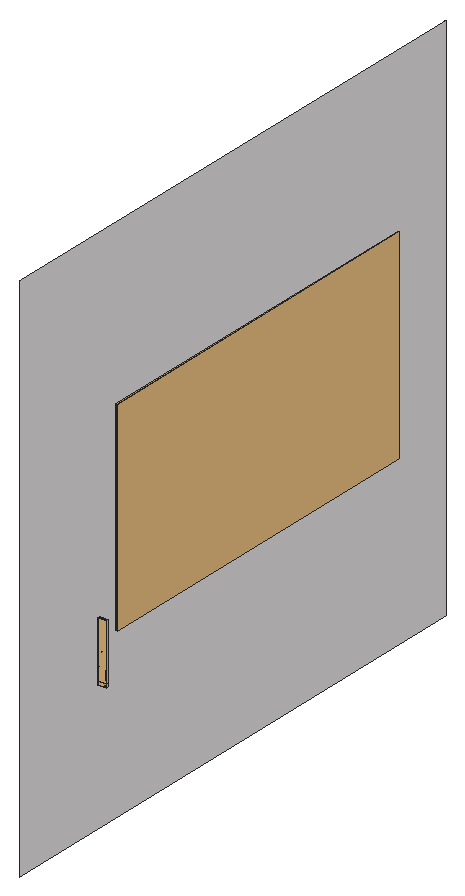
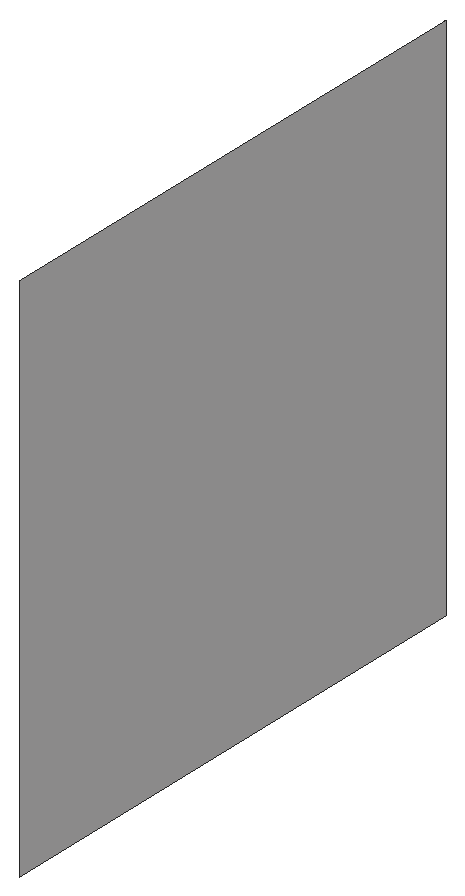
# SketchUp Ruby script. Lengths in inches.
U = 1.inch
M = Sketchup.active_model
def pt(a) = Geom::Point3d.new(a.map { |v| v * U })
def face(e, loops, mat)
  f = e.add_face(loops[0].map { |a| pt(a) })
  loops[1..].each { |l| e.add_face(l.map { |a| pt(a) }).erase! }
  f.material = f.back_material = mat if mat
  f
end
# faces: each face lists its corners as indices into pts; further lists are holes
def faces(e, pts, list, mat = nil) = list.each { |f| face(e, (f[0].is_a?(Array) ? f : [f]).map { |l| l.map { |i| pts[i] } }, mat) }
# xy, xz, yz: faces in a plane at the given z, y or x. An outline is a flat list of corners, or four numbers for a rectangle; further outlines are holes
def ring(l) = l.size == 4 ? [[l[0], l[1]], [l[2], l[1]], [l[2], l[3]], [l[0], l[3]]] : l.each_slice(2).to_a
def flat(e, list, mat, &to3) = list.each { |f| face(e, (f[0].is_a?(Array) ? f : [f]).map { |l| ring(l).map { |u, v| to3.(u, v) } }, mat) }
def xy(e, z, list, mat = nil) = flat(e, list, mat) { |x, y| [x, y, z] }
def xz(e, y, list, mat = nil) = flat(e, list, mat) { |x, z| [x, y, z] }
def yz(e, x, list, mat = nil) = flat(e, list, mat) { |y, z| [x, y, z] }
def lines(e, pts, list) = list.each { |a, b| e.add_line(pt(pts[a]), pt(pts[b])) }
# prism: a flat outline (further loops are holes) pulled along v
def prism(e, loops, v, mat = nil)
  f = face(e, loops, mat); d = Geom::Vector3d.new(v.map { |x| x * U })
  f.pushpull(f.normal.samedirection?(d) ? d.length : -d.length)
end
def box(e, o, s, mat = nil) = prism(e, [[o, [o[0] + s[0], o[1], o[2]], [o[0] + s[0], o[1] + s[1], o[2]], [o[0], o[1] + s[1], o[2]]]], [0, 0, s[2]], mat)
def at(x, y, z, deg = 0) = Geom::Transformation.translation(pt([x, y, z])) * Geom::Transformation.rotation(ORIGIN, Z_AXIS, deg.degrees)
def axes(o, x, y, z) = Geom::Transformation.new([*x, 0, *y, 0, *z, 0, *pt(o).to_a, 1])
def part(name) = M.definitions.add(name)
# library, detail: a bought-in or finely detailed component or shape, given as its bounding box
def library(name, o, s) = part(name).tap { |d| box(d.entities, o, s) }
def detail(e, o, s) = box(e.add_group.entities, o, s)
def put(e, d, t, mat = nil) = e.add_instance(d, t).tap { |i| i.material = mat if mat }
def group(e, t, mat = nil) = e.add_group.tap { |g| g.transformation = t; g.material = mat if mat }.entities
root = M.entities
M.materials.add("[Stone Vein Gray]").color = [225, 223, 223]
M.materials.add("green").color = [174, 139, 102]
M.materials.add("vio").color = [206, 114, 100]
c1 = library("3DGeom~133_Defintion",[-19.91,-529.75,-72.32],[39.82,1000,144.37])
c2 = library("3DGeom~131_Defintion",[-19.41,-483.5625,-70.5],[38.82,1000,140.74])
c3 = part("3DGeom~134_Defintion")
p = [[-9.17,365.0625,-60.44],[-10.66,319.24,-60.24],[-9.24,319.23,-61.125],[-10.63,365.04,-59.53],[-12.34,365.04,-59.02],[-14.12,365.04,-58.98],
  [-14.05,319.22,-59.71],[-12.32,319.23,-59.75],[-8.56,277.89,-58.6875],[-8.45,241.12,-52.31],[-7.11,241.05,-53.13],[-9.93,277.92,-57.83],
  [-11.54,277.92,-57.36],[-13.22,277.89,-57.32],[-11.63,241.07,-51.81],[-10.01,241.13,-51.85],[-6.75,470.15,-49.68],[-9.84,415.33,-55.7],
  [-8.34,415.37,-56.63],[-8.29,470.08,-48.72],[-10.1,470.07,-48.1875],[-13.43,415.34,-55.13],[-11.6,415.32,-55.17],[-11.98,470.11,-48.14],
  [-4.1,211.43,-41.85],[-0.64,188.37,-23.41],[0.67,188.13,-24.11],[-5.42,211.6,-41.08],[-6.95,211.62,-40.63],[-8.53,211.47,-40.56],
  [-3.6875,188.18,-22.85],[-2.14,188.39,-22.97],[6.29,168.75,-2.9375],[10.49,151.32,19.02],[11.76,151.06,18.38],[6.29,168.75,-2.9375],
  [4.99,169.02,-2.29],[10.49,151.32,19.02],[3.51,169.05,-1.87],[2,168.82,-1.72],[7.55,151.14,19.55],[9.03,151.35,19.42],
  [-2.58,-7.65,9.24],[-5.6,-27.13,7.79],[-4.52,-27.2,7.15],[-3.69,-7.65,9.88],[-4.97,-7.58,10.22],[-6.28,-7.43,10.23],
  [-8.15,-27.06,8.11],[-6.85,-27.08,8.125],[-3.875,-43.53,12.625],[-2.45,-57.47,24.41],[-1.39,-57.67,23.87],[-4.94,-43.36,13.22],
  [-6.17,-43.32,13.55],[-7.45,-43.42,13.58],[-4.9,-57.59,24.83],[-3.66,-57.4375,24.75],[7.01,37.63,28.93],[0.5,14.23,18.1875],
  [1.64,14.26,17.55],[5.85,37.59,29.58],[4.53,37.68,29.94],[-2.125,14.51,18.57],[-0.8,14.3125,18.55],[3.18,37.89,29.97],
  [5.56,-294.46,30.13],[4.07,-328.71,26.72],[4.85,-328.71,26.23],[4.75,-294.51,30.64],[4.86,-362.1,26.86],[4.11,-362.08,27.33],
  [4.47,-395.52,30.27],[5.1875,-395.55,29.82],[3.8,-294.53,30.93],[2.8125,-294.51,30.96],[2.21,-328.71,27.03],[3.16,-328.71,27],
  [3.23,-362.08,27.6],[2.32,-362.08,27.63],[2.75,-395.51,30.56],[3.63,-395.5,30.53],[5.84,-429.05,35.11],[6.16,-462.54,43.14],
  [6.82,-462.6,42.73],[5.15,-429,35.54],[4.35,-428.98,35.79],[3.51,-428.99,35.8125],[4.58,-462.53,43.4],[5.39,-462.51,43.375],
  [16.05,132.58,36.39],[16.75,110.79,47.79],[17.95,110.68,47.08],[14.8125,132.8,37.06],[13.38,132.84,37.45],[11.91,132.69,37.51],
  [13.89,110.82,48.16],[15.34,110.84,48.16],[2.27,-71.39,38.47],[5.25,-86.23,54.01],[6.27,-86.4,53.46],[1.23,-71.18,39],
  [8.9,-222.87,50.33],[6.22,-258.8,39.57],[7.0625,-258.72,39.05],[0.04,-71.16,39.34],[-1.17,-71.33,39.4375],[2.89,-86.37,54.44],
  [4.09,-86.22,54.36],[8.03,-222.96,50.86],[7.01,-223,51.17],[5.95,-222.97,51.21],[4.22,-258.8,39.9],[5.24,-258.83,39.86],
  [16.42,86.25,47.3],[11.16,61.76,40.67],[12.34,61.78,40],[15.23,86.27,48],[13.86,86.35,48.37],[8.43,62.04,41.06],
  [9.8125,61.85,41.04],[12.44,86.47,48.36],[8.12,-496.2,52.69],[9.15,-529.77,65.34],[9.75,-529.85,64.98],[7.49,-496.125,53.08],
  [6.76,-496.1,53.3],[5.99,-496.12,53.32],[7.72,-529.76,65.58],[8.45,-529.74,65.55],[11.66,-156.24,69.3],[9.6875,-188.37,61.86],
  [10.59,-188.28,61.31],[10.73,-156.3,69.88],[9.64,-156.33,70.21],[8.51,-156.32,70.24],[7.54,-188.38,62.22],[8.64,-188.4,62.18],
  [9.71,-104.66,65.64],[8.72,-104.5625,66.23],[10.65,-127.92,72.15],[11.61,-127.92,71.55],[7.58,-104.56,66.57],[6.4,-104.66,66.625],
  [8.36,-127.96,72.52],[9.53,-127.93,72.49]]
faces(c3.entities,p,[[0,1,2],[0,3,1],[4,5,6],[4,6,7],[8,9,10],[8,11,9],[12,13,14],[12,14,15],
  [16,17,18],[16,19,17],[20,21,22],[20,23,21],[24,25,26],[24,27,25],[28,29,30],[28,30,31],
  [32,33,34],[35,36,37],[38,39,40],[38,40,41],[42,43,44],[42,45,43],[46,47,48],[46,48,49],
  [50,51,52],[50,53,51],[54,55,56],[54,56,57],[58,59,60],[58,61,59],[62,63,64],[62,65,63],
  [66,67,68],[66,69,67],[70,71,72],[70,72,73],[74,75,76],[74,76,77],[78,79,80],[78,80,81],
  [82,83,84],[82,85,83],[86,87,88],[86,88,89],[90,91,92],[90,93,91],[94,95,96],[94,96,97],
  [98,99,100],[98,101,99],[102,103,104],[105,106,107],[105,107,108],[102,109,103],[110,111,112],[110,112,113],
  [114,115,116],[114,117,115],[118,119,120],[118,121,119],[122,123,124],[122,125,123],[126,127,128],[126,128,129],
  [130,131,132],[130,133,131],[134,135,136],[134,136,137],[138,139,140],[138,140,141],[142,143,144],[142,144,145]],"green")
c4 = part("3DGeom~132_Defintion")
p = [[-9.01,311.27,-59.6],[-10.4,311.27,-58.74],[-9.6875,270.99,-56.39],[-8.34,270.95,-57.22],[-8.13,405.01,-55.22],[-10.37,355.9375,-58.05],
  [-8.94,355.96,-58.93],[-12.01,311.27,-58.26],[-13.69,311.26,-58.22],[-12.89,270.96,-55.89],[-11.25,270.99,-55.92],[-9.6,404.97,-54.31],
  [-11.31,404.95,-53.8],[-13.77,355.9375,-57.51],[-12.03,355.93,-57.55],[-13.1,404.98,-53.75],[-6.9375,235.04,-51.81],[-5.28,206.32,-40.06],
  [-3.99,206.16,-40.81],[-8.24,235.11,-51],[-9.76,235.11,-50.55],[-11.34,235.05,-50.51],[-8.32,206.19,-39.54],[-6.77,206.34,-39.62],
  [-4.28,516.18,-38.61],[-8.09,458.36,-47.51],[-6.58,458.42,-48.44],[-5.83,516.1,-37.65],[-7.64,516.08,-37.11],[-11.68,458.38,-46.9375],
  [-9.85,458.34,-46.98],[-9.53,516.13,-37.0625],[0.66,183.44,-23.51],[4.86,164.8,-2.23],[6.13,164.54,-2.87],[-0.625,183.67,-22.83],
  [-2.09,183.69,-22.4],[-3.59,183.49,-22.28],[1.95,164.61,-1.68],[3.42,164.83,-1.82],[-4.41,-26.52,6.97],[-4.82,-42.28,12.89],
  [-3.78,-42.44,12.31],[-5.46,-26.45,7.59],[-6.68,-26.4,7.92],[-7.95,-26.38,7.91],[-7.26,-42.34,13.24],[-6.02,-42.24,13.21],
  [1.59,13.9,17.11],[-3.6,-7.46,9.63],[-2.52,-7.46,9.01],[0.49,13.87,17.73],[-0.78,13.96,18.08],[-6.12,-7.25,9.97],
  [-4.84,-7.39,9.97],[-2.07,14.15,18.11],[11.47,147.29,17.92],[14.44,129.49,36.13],[15.65,129.27,35.48],[11.47,147.29,17.92],
  [10.22,147.54,18.54],[8.81,147.58,18.9375],[7.36,147.375,19.06],[11.62,129.38,36.57],[13.05,129.53,36.51],[-1.35,-56.24,23.27],
  [1.2,-69.4,38.03],[2.21,-69.6,37.51],[-2.38,-56.03,23.8],[-3.5625,-56,24.13],[-4.77,-56.16,24.21],[-1.15,-69.55,38.45],
  [0.04,-69.38,38.36],[4.73,-320.51,25.58],[3.97,-320.51,26.06],[4.01,-353.05,26.65],[4.74,-353.07,26.19],[3.08,-320.51,26.33],
  [2.15,-320.51,26.36],[2.26,-353.05,26.94],[3.15,-353.05,26.91],[12.03,60.24,39],[5.7,36.65,28.84],[6.83,36.6875,28.21],
  [10.88,60.22,39.65],[5.06,-385.68,29.08],[4.36,-385.65,29.52],[5.02,-418.3,34.66],[5.7,-418.34,34.23],[9.57,60.3,40.01],
  [3.1,36.95,29.23],[4.41,36.74,29.2],[8.22,60.49,40.03],[6.89,-252.26,38.07],[4.63,-287.17,29.875],[5.42,-287.12,29.38],
  [3.54,-385.64,29.77],[2.68,-385.64,29.79],[3.42,-418.29,34.92],[4.24,-418.28,34.89],[6.07,-252.34,38.58],[5.11,-252.37,38.87],
  [4.11,-252.34,38.9],[2.74,-287.17,30.1875],[3.71,-287.19,30.16],[6.65,-451.06,41.67],[7.3,-483.75,51.75],[7.92,-483.82,51.375],
  [6.01,-451,42.07],[5.26,-450.97,42.29],[4.47,-450.99,42.32],[5.84,-483.74,51.99],[6.59,-483.72,51.97],[17.5,107.92,45.9],
  [16.33,108.02,46.59],[14.85,84.12,46.8],[16.01,84.1,46.12],[14.96,108.07,46.96],[12.125,84.32,47.16],[13.51,84.19,47.16],
  [13.54,108.06,46.96],[10.32,-183.58,59.78],[7.83,-217.4,49.6],[8.67,-217.31,49.07],[9.44,-183.67,60.32],[8.42,-183.7,60.63],
  [7.35,-183.68,60.66],[5.8,-217.4,49.93],[6.83,-217.43,49.89],[6.11,-84.25,52.125],[8.51,-101.95,64.58],[9.47,-102.05,64],
  [5.12,-84.08,52.67],[3.99,-84.07,53],[2.82,-84.22,53.08],[6.24,-102.05,64.96],[7.39,-101.95,64.91],[11.32,-124.73,69.76],
  [10.46,-152.4,68.13],[11.37,-152.34,67.57],[10.39,-124.73,70.35],[9.3,-124.74,70.69],[8.15,-124.76,70.71],[8.29,-152.42,68.49],
  [9.4,-152.43,68.46]]
faces(c4.entities,p,[[0,1,2],[0,2,3],[4,5,6],[7,8,9],[7,9,10],[4,11,5],[12,13,14],[12,15,13],
  [16,17,18],[16,19,17],[20,21,22],[20,22,23],[24,25,26],[24,27,25],[28,29,30],[28,31,29],
  [32,33,34],[32,35,33],[36,37,38],[36,38,39],[40,41,42],[40,43,41],[44,45,46],[44,46,47],
  [48,49,50],[48,51,49],[52,53,54],[52,55,53],[56,57,58],[59,60,57],[61,62,63],[61,63,64],
  [65,66,67],[65,68,66],[69,70,71],[69,71,72],[73,74,75],[73,75,76],[77,78,79],[77,79,80],
  [81,82,83],[81,84,82],[85,86,87],[85,87,88],[89,90,91],[89,92,90],[93,94,95],[96,97,98],
  [96,98,99],[93,100,94],[101,102,103],[101,103,104],[105,106,107],[105,108,106],[109,110,111],[109,111,112],
  [113,114,115],[113,115,116],[117,118,119],[117,120,118],[121,122,123],[121,124,122],[125,126,127],[125,127,128],
  [129,130,131],[129,132,130],[133,134,135],[133,135,136],[137,138,139],[137,140,138],[141,142,143],[141,143,144]],"green")
c5 = part("3DGeom~130_Defintion")
p = [[-10.63,365.1,-59.54],[-12.32,319.28,-59.76],[-10.66,319.28,-60.25],[-12.34,365.09,-59.03],[-9.9375,277.96,-57.84],[-11.54,277.96,-57.36],
  [-10.01,241.16,-51.85],[-8.45,241.16,-52.32],[-8.3,470.15,-48.73],[-11.6,415.375,-55.18],[-9.85,415.39,-55.7],[-10.1,470.14,-48.19],
  [-5.42,211.63,-41.09],[-6.95,211.65,-40.64],[-2.14,188.42,-22.97],[-0.64,188.4,-23.41],[4.99,169.04,-2.29],[9.03,151.375,19.43],
  [10.49,151.34,19.02],[3.51,169.07,-1.87],[-3.69,-7.65,9.88],[-6.85,-27.08,8.125],[-5.6,-27.13,7.79],[-4.97,-7.58,10.23],
  [-4.94,-43.37,13.22],[-3.66,-57.45,24.75],[-2.45,-57.48,24.42],[-6.18,-43.33,13.55],[5.85,37.6,29.58],[-0.8,14.32,18.55],
  [0.5,14.23,18.19],[4.53,37.6875,29.95],[4.75,-294.56,30.64],[3.16,-328.76,27.01],[4.07,-328.76,26.73],[3.8,-294.58,30.93],
  [4.11,-362.14,27.34],[3.23,-362.13,27.61],[3.63,-395.56,30.53],[4.47,-395.57,30.28],[5.15,-429.0625,35.55],[4.35,-429.04,35.79],
  [5.39,-462.58,43.38],[6.16,-462.6,43.15],[14.8125,132.82,37.06],[15.35,110.85,48.17],[16.75,110.8,47.79],[13.39,132.86,37.45],
  [1.23,-71.19,39],[0.04,-71.17,39.34],[4.09,-86.23,54.36],[5.25,-86.24,54.02],[8.03,-222.99,50.87],[5.24,-258.86,39.87],
  [6.22,-258.83,39.57],[7.01,-223.03,51.18],[15.23,86.29,48],[9.81,61.86,41.04],[11.16,61.77,40.67],[13.86,86.36,48.375],
  [7.49,-496.2,53.08],[6.76,-496.17,53.3],[8.45,-529.82,65.5625],[9.15,-529.85,65.35],[10.73,-156.33,69.89],[8.64,-188.43,62.1875],
  [9.6875,-188.39,61.87],[9.64,-156.35,70.22],[8.73,-104.58,66.24],[7.58,-104.57,66.58],[9.53,-127.95,72.5],[10.66,-127.9375,72.16]]
faces(c5.entities,p,[[0,1,2],[0,3,1],[4,5,6],[4,6,7],[8,9,10],[8,11,9],[12,13,14],[12,14,15],
  [16,17,18],[16,19,17],[20,21,22],[20,23,21],[24,25,26],[24,27,25],[28,29,30],[28,31,29],
  [32,33,34],[32,35,33],[36,37,38],[36,38,39],[40,41,42],[40,42,43],[44,45,46],[44,47,45],
  [48,49,50],[48,50,51],[52,53,54],[52,55,53],[56,57,58],[56,59,57],[60,61,62],[60,62,63],
  [64,65,66],[64,67,65],[68,69,70],[68,70,71]],"green")
c6 = part("3DGeom~129_Defintion")
p = [[-10.4,311.32,-58.75],[-12.01,311.32,-58.27],[-11.25,271.03,-55.93],[-9.6875,271.03,-56.4],[-9.6,405.03,-54.31],[-12.03,355.98,-57.5625],
  [-10.37,355.99,-58.06],[-11.3125,405.02,-53.8],[-8.24,235.14,-51.01],[-9.76,235.15,-50.5625],[-6.78,206.37,-39.62],[-5.28,206.35,-40.0625],
  [-5.83,516.18,-37.66],[-9.85,458.41,-46.99],[-8.09,458.42,-47.52],[-7.64,516.16,-37.12],[-0.625,183.7,-22.83],[3.42,164.86,-1.82],
  [4.87,164.83,-2.23],[-2.09,183.72,-22.4],[-5.46,-26.46,7.59],[-6.68,-26.41,7.92],[-6.02,-42.25,13.22],[-4.82,-42.29,12.89],
  [0.49,13.875,17.74],[-4.84,-7.39,9.97],[-3.6,-7.46,9.63],[-0.78,13.96,18.09],[10.23,147.57,18.54],[8.81,147.6,18.94],
  [13.05,129.54,36.52],[14.44,129.5,36.14],[-2.39,-56.04,23.81],[-3.56,-56.01,24.13],[0.04,-69.39,38.36],[1.2,-69.42,38.03],
  [3.97,-320.56,26.0625],[3.08,-320.5625,26.33],[3.15,-353.1,26.92],[4.01,-353.11,26.65],[10.88,60.23,39.66],[4.41,36.75,29.2],
  [5.7,36.66,28.85],[9.57,60.3125,40.02],[4.36,-385.71,29.52],[4.24,-418.34,34.9],[5.02,-418.36,34.66],[3.54,-385.69,29.77],
  [6.07,-252.38,38.58],[3.71,-287.23,30.16],[4.63,-287.21,29.88],[5.11,-252.41,38.875],[6.01,-451.07,42.07],[5.26,-451.04,42.3],
  [6.59,-483.8,51.97],[7.31,-483.82,51.76],[16.33,108.04,46.6],[13.51,84.21,47.17],[14.85,84.13,46.81],[14.96,108.09,46.97],
  [9.45,-183.7,60.33],[6.84,-217.47,49.9],[7.83,-217.43,49.6],[8.42,-183.73,60.64],[5.12,-84.09,52.67],[3.99,-84.08,53.01],
  [7.39,-101.97,64.92],[8.51,-101.97,64.59],[10.39,-124.75,70.36],[9.4,-152.46,68.47],[10.46,-152.43,68.15],[9.3,-124.76,70.7]]
faces(c6.entities,p,[[0,1,2],[0,2,3],[4,5,6],[4,7,5],[8,9,10],[8,10,11],[12,13,14],[12,15,13],
  [16,17,18],[16,19,17],[20,21,22],[20,22,23],[24,25,26],[24,27,25],[28,29,30],[28,30,31],
  [32,33,34],[32,34,35],[36,37,38],[36,38,39],[40,41,42],[40,43,41],[44,45,46],[44,47,45],
  [48,49,50],[48,51,49],[52,53,54],[52,54,55],[56,57,58],[56,59,57],[60,61,62],[60,63,61],
  [64,65,66],[64,66,67],[68,69,70],[68,71,69]],"green")
c7 = part("3DGeom~212_Defintion")
p = [[-253.96,-102.22,-418.25],[-4.58,-88.53,-492.98],[51.95,-256.53,-399.89],[278.67,-148.1,-381.875],[51.95,-256.53,-399.89],[246.04,-51.11,-435.625],
  [-251.19,119.16,-413.67],[-253.96,-102.22,-418.25],[-251.19,119.16,-413.67],[-2.17,103.2,-489.02],[247.42,59.58,-433.34],[58.52,267.27,-389.07],
  [-181.11,308.61,-298.26],[-251.19,119.16,-413.67],[-181.11,308.61,-298.26],[278.67,-148.1,-381.875],[246.04,-51.11,-435.625],[430.72,0,-261.54],
  [430.72,0,-261.54],[247.42,59.58,-433.34],[282.46,154.31,-375.63],[282.46,154.31,-375.63],[-435.3,-88.53,-231.44],[-253.96,-102.22,-418.25],
  [-188.69,-296.21,-310.75],[-253.96,-102.22,-418.25],[51.95,-256.53,-399.89],[-188.69,-296.21,-310.75],[-432.9,103.2,-227.48],[-251.19,119.16,-413.67],
  [-372.21,267.26,-127.53],[-181.11,308.61,-298.26],[-188.69,-296.21,-310.75],[51.95,-256.53,-399.89],[152.27,-355.79,-234.68],[51.95,-256.53,-399.89],
  [336.59,-205.41,-286.49],[152.27,-355.79,-234.68],[51.95,-256.53,-399.89],[336.59,-205.41,-286.49],[161.24,359.72,-219.91],[-62.5,415.37,-102.93],
  [58.52,267.27,-389.07],[-181.11,308.61,-298.26],[161.24,359.72,-219.91],[58.52,267.27,-389.07],[336.59,-205.41,-286.49],[278.67,-148.1,-381.875],
  [282.46,154.31,-375.63],[341.77,207.68,-277.97],[161.24,359.72,-219.91],[341.77,207.68,-277.97],[-378.77,-256.53,-138.34],[-72.86,-410.83,-119.99],
  [-188.69,-296.21,-310.75],[-378.77,-256.53,-138.34],[-269.49,359.72,41.63],[-181.11,308.61,-298.26],[-372.21,267.26,-127.53],[-269.49,359.72,41.63],
  [-181.11,308.61,-298.26],[336.59,-205.41,-286.49],[404.27,-207.68,-175.04],[404.27,-207.68,-175.04],[336.59,-205.41,-286.49],[341.77,207.68,-277.97],
  [409.45,205.41,-166.51],[278.46,355.79,-26.86],[409.45,205.41,-166.51],[341.77,207.68,-277.97],[341.77,207.68,-277.97],[463.57,-154.31,-77.37],
  [498.61,-59.58,-19.66],[500,51.11,-17.38],[409.45,205.41,-166.51],[467.36,148.11,-71.13],[269.49,-359.72,-41.63],[404.27,-207.68,-175.04],
  [-500,-51.11,17.38],[-498.61,59.58,19.66],[-463.57,154.3,77.37],[72.86,410.83,119.98],[269.49,-359.72,-41.63],[378.77,256.53,138.34],
  [409.45,205.41,-166.51],[378.77,256.53,138.34],[409.45,205.41,-166.51],[278.46,355.79,-26.86],[-378.77,-256.53,-138.34],[-278.46,-355.79,26.86],
  [-467.36,-148.11,71.13],[-278.46,-355.79,26.86],[-404.27,207.68,175.04],[-269.49,359.72,41.63],[62.5,-415.37,102.93],[-152.27,355.79,234.68],
  [-269.49,359.72,41.63],[269.49,-359.72,-41.63],[372.21,-267.27,127.53],[435.3,88.53,231.44],[378.77,256.53,138.34],[372.21,-267.27,127.53],
  [188.69,296.21,310.75],[378.77,256.53,138.34],[432.9,-103.2,227.48],[-430.72,0,261.54],[-161.24,-359.72,219.91],[-409.45,-205.41,166.51],
  [-161.24,-359.72,219.91],[-278.46,-355.79,26.86],[-409.45,-205.41,166.51],[-336.59,205.41,286.49],[-269.49,359.72,41.63],[-404.27,207.68,175.04],
  [-336.59,205.41,286.49],[-269.49,359.72,41.63],[-161.24,-359.72,219.91],[181.11,-308.61,298.26],[372.21,-267.27,127.53],[181.11,-308.61,298.26],
  [-51.95,256.53,399.89],[-51.95,256.53,399.89],[181.11,-308.61,298.26],[253.96,102.22,418.25],[378.77,256.53,138.34],[253.96,102.22,418.25],
  [378.77,256.53,138.34],[188.69,296.21,310.75],[-409.45,-205.41,166.51],[-161.24,-359.72,219.91],[-341.77,-207.68,277.97],[-341.77,-207.68,277.97],
  [-336.59,205.41,286.49],[-341.77,-207.68,277.97],[-161.24,-359.72,219.91],[-58.52,-267.27,389.07],[-161.24,-359.72,219.91],[181.11,-308.61,298.26],
  [-58.52,-267.27,389.07],[181.11,-308.61,298.26],[251.1875,-119.16,413.67],[251.1875,-119.16,413.67],[251.1875,-119.16,413.67],[253.96,102.22,418.25],
  [-278.67,148.1,381.875],[-152.27,355.79,234.68],[-336.59,205.41,286.49],[-278.67,148.1,381.875],[-51.95,256.53,399.89],[-152.27,355.79,234.68],
  [-282.46,-154.31,375.63],[-247.42,-59.58,433.34],[-247.42,-59.58,433.34],[-246.04,51.11,435.625],[-430.72,0,261.54],[-278.67,148.1,381.875],
  [-246.04,51.11,435.625],[-341.77,-207.68,277.97],[-282.46,-154.31,375.63],[181.11,-308.61,298.26],[251.1875,-119.16,413.67],[4.58,88.53,492.98],
  [188.69,296.21,310.75],[253.96,102.22,418.25],[188.69,296.21,310.75],[-282.46,-154.31,375.63],[2.17,-103.2,489.02],[-282.46,-154.31,375.63],
  [-247.42,-59.58,433.34],[-246.04,51.11,435.625],[-278.67,148.1,381.875],[-246.04,51.11,435.625],[-247.42,-59.58,433.34],[-247.42,-59.58,433.34],
  [-246.04,51.11,435.625]]
faces(c7.entities,p,[[0,1,2],[1,3,4],[1,5,3],[6,1,7],[8,9,1],[9,5,1],[9,10,5],[11,10,9],
  [12,9,13],[14,11,9],[15,16,17],[5,10,18],[19,20,17],[11,21,10],[22,23,24],[25,26,27],
  [28,23,22],[28,29,23],[30,29,28],[30,31,29],[32,33,34],[35,36,37],[38,3,39],[40,21,11],
  [41,42,43],[41,44,45],[46,47,17],[48,49,17],[50,51,21],[52,32,53],[32,34,53],[22,54,55],
  [56,57,58],[59,41,60],[34,61,62],[63,64,17],[65,66,17],[67,68,69],[67,70,44],[71,63,17],
  [72,71,17],[73,72,17],[74,75,17],[75,73,17],[53,34,76],[34,77,76],[78,22,55],[79,22,78],
  [79,28,22],[80,28,79],[80,30,28],[81,67,44],[81,44,41],[82,63,71],[83,75,84],[85,86,87],
  [88,53,89],[90,55,91],[78,55,90],[92,30,80],[92,93,30],[89,53,94],[53,76,94],[95,41,96],
  [95,81,41],[97,71,98],[98,71,72],[99,73,75],[99,75,100],[94,76,101],[102,103,67],[102,67,81],
  [98,72,104],[104,72,73],[104,73,99],[78,90,105],[79,78,105],[80,79,105],[89,94,106],[107,89,108],
  [90,109,110],[111,112,113],[114,95,115],[90,110,105],[92,80,105],[116,94,117],[94,118,119],[120,81,95],
  [121,102,81],[122,98,104],[123,99,124],[125,126,127],[128,129,130],[110,131,105],[132,92,105],[133,134,135],
  [136,137,138],[139,104,140],[141,104,99],[142,99,143],[144,145,146],[147,148,149],[131,150,105],[150,151,105],
  [152,153,154],[155,132,105],[156,155,105],[157,135,158],[135,159,160],[161,162,148],[161,163,164],[165,135,166],
  [167,166,168],[169,148,170],[135,160,166],[171,161,148],[166,160,163],[166,163,161],[172,166,161],[173,161,174]],"vio")
c8 = library("3DGeom~146_Defintion",[-500,-464.96,-145.56],[1000,929.92,291.12])
c9 = part("3DGeom~147_Defintion")
p = [[447.11,-464.11,-119.78],[466.43,-447.31,-145.56],[454.24,-459.97,-82.98],[466.43,-447.31,-145.56],[447.11,-464.11,-119.78],[454.17,-457.65,-136.37],
  [454.24,-459.97,-82.98],[466.43,-447.31,-145.56],[480.68,-439.04,-71.95],[466.43,-447.31,-145.56],[480.59,-435.86,-144.88],[492.87,-426.375,-134.53],
  [500,-422.24,-97.72],[466.43,-447.31,-145.56],[492.87,-426.375,-134.53],[480.68,-439.04,-71.95],[466.43,-447.31,-145.56],[492.87,-426.375,-134.53],
  [499.98,-421.39,-117.27],[447.11,-464.11,-119.78],[454.24,-459.97,-82.98],[447.13,-464.96,-100.24],[480.68,-439.04,-71.95],[492.9375,-428.7,-81.14],
  [454.24,-459.97,-82.98],[480.68,-439.04,-71.95],[466.52,-450.48,-72.62],[-486.65,450.01,82.87],[-454.24,464.96,91.16],[-470.88,459.85,82.8125],
  [-486.65,450.01,82.87],[-494.01,420.39,122.7],[-480.9375,419.38,137.21],[-486.65,450.01,82.87],[-480.9375,419.38,137.21],[-464.29,424.49,145.56],
  [-486.65,450.01,82.87],[-500,427.23,105.9],[-494.01,420.39,122.7],[-486.65,450.01,82.87],[-464.29,424.49,145.56],[-448.53,434.33,145.5],
  [-486.65,450.01,82.87],[-497.31,438.07,91.32],[-500,427.23,105.9],[-486.65,450.01,82.87],[-448.53,434.33,145.5],[-437.87,446.27,137.04],
  [-486.65,450.01,82.87],[-437.87,446.27,137.04],[-435.17,457.12,122.47],[-486.65,450.01,82.87],[-441.17,463.96,105.67],[-454.24,464.96,91.16],
  [-486.65,450.01,82.87],[-435.17,457.12,122.47]]
faces(c9.entities,p,[[0,1,2],[3,4,5],[6,7,8],[9,10,11],[12,13,14],[15,16,12],[12,17,18],[19,20,21],
  [22,12,23],[24,25,26],[27,28,29],[30,31,32],[33,34,35],[36,37,38],[39,40,41],[42,43,44],
  [45,46,47],[48,49,50],[51,52,53],[54,55,52]],"green")
c10 = part("3DGeom~235_Defintion")
p = [[111.34,-218.38,-429.9],[-247.29,-210.43,-375.22],[-78.46,-72.24,-500],[275.78,-41.25,-430.1],[-393.46,-67.1,-319.9],[-393.46,-67.1,-319.9],
  [-247.23,93.26,-436.12],[111.4,85.3125,-490.8],[366.3125,146.93,-315.04],[-34.76,228.64,-435.48],[271.41,220,-350.09],[366.3125,146.93,-315.04],
  [271.41,220,-350.09],[-247.23,93.26,-436.12],[-393.46,-67.1,-319.9],[-482.25,54.59,-163.38],[-247.23,93.26,-436.12],[-349.76,233.77,-255.38],
  [-349.76,233.77,-255.38],[271.41,220,-350.09],[187.03,302.75,-318.15],[-349.76,233.77,-255.38],[-123.56,350.33,-278.96],[187.03,302.75,-318.15],
  [-123.56,350.33,-278.96],[414.31,-117.14,-269.63],[446.3,103.11,-222.4],[414.31,-117.14,-269.63],[275.78,-41.25,-430.1],[275.78,-41.25,-430.1],
  [366.3125,146.93,-315.04],[-82.92,-337,-314.52],[271.31,-306.01,-244.62],[-82.92,-337,-314.52],[111.34,-218.38,-429.9],[414.31,-117.14,-269.63],
  [271.31,-306.01,-244.62],[-82.92,-337,-314.52],[-349.87,-292.24,-149.91],[-247.29,-210.43,-375.22],[-247.29,-210.43,-375.22],[-349.87,-292.24,-149.91],
  [-434.26,-209.49,-117.97],[-247.29,-210.43,-375.22],[271.41,220,-350.09],[358.7,295.74,-115.58],[187.03,302.75,-318.15],[-485.52,-139.23,-27.6],
  [187.03,302.75,-318.15],[135.76,373.01,-227.78],[358.7,295.74,-115.58],[187.03,302.75,-318.15],[-123.56,350.33,-278.96],[135.76,373.01,-227.78],
  [55.61,-412.89,-154.05],[-254.97,-365.3125,-114.86],[-82.92,-337,-314.52],[271.31,-306.01,-244.62],[-82.92,-337,-314.52],[-82.92,-337,-314.52],
  [-349.87,-292.24,-149.91],[-123.56,350.33,-278.96],[-349.76,233.77,-255.38],[-358.58,311.65,-6.22],[-131.1875,417.76,-63.17],[489.89,-122.02,-52.4],
  [271.31,-306.01,-244.62],[489.93,100.3,-96.98],[-349.76,233.77,-255.38],[-489.89,122.02,52.4],[-349.76,233.77,-255.38],[-358.58,311.65,-6.22],
  [358.58,-311.65,6.22],[271.31,-306.01,-244.62],[358.58,-311.65,6.22],[271.31,-306.01,-244.62],[131.35,411.94,-103.2],[358.7,295.74,-115.58],
  [-489.93,-100.3,96.98],[131.1875,-417.76,63.17],[-174.99,-409.125,-22.22],[358.58,-311.65,6.22],[-254.97,-365.3125,-114.86],[-358.7,-295.74,115.58],
  [-358.7,-295.74,115.58],[-358.7,-295.74,115.58],[485.52,139.23,27.6],[434.26,209.49,117.97],[349.87,292.24,149.91],[254.97,365.3125,114.86],
  [174.99,409.125,22.22],[358.7,295.74,-115.58],[254.97,365.3125,114.86],[358.7,295.74,-115.58],[-358.7,-295.74,115.58],[-55.61,412.89,154.05],
  [-271.31,306.01,244.62],[482.25,-54.59,163.38],[-358.7,-295.74,115.58],[-131.35,-411.94,103.2],[-358.58,311.65,-6.22],[-414.31,117.14,269.63],
  [-358.58,311.65,-6.22],[-414.31,117.14,269.63],[-271.31,306.01,244.62],[349.76,-233.77,255.39],[358.58,-311.65,6.22],[349.76,-233.77,255.39],
  [82.92,337,314.52],[254.97,365.3125,114.86],[-446.3,-103.11,222.4],[-414.31,117.14,269.63],[123.56,-350.33,278.96],[349.76,-233.77,255.39],
  [-358.7,-295.74,115.58],[-135.76,-373.01,227.78],[254.97,365.3125,114.86],[247.29,210.43,375.22],[254.97,365.3125,114.86],[247.29,210.43,375.22],
  [349.87,292.24,149.91],[-187.03,-302.75,318.15],[-187.03,-302.75,318.15],[-271.41,-220,350.09],[-358.7,-295.74,115.58],[-366.31,-146.93,315.04],
  [-358.7,-295.74,115.58],[-271.41,-220,350.09],[-366.31,-146.93,315.04],[-358.7,-295.74,115.58],[393.46,67.1,319.9],[247.29,210.43,375.22],
  [-111.34,218.38,429.9],[-111.34,218.38,429.9],[-414.31,117.14,269.63],[-366.31,-146.93,315.04],[34.76,-228.64,435.48],[-187.03,-302.75,318.15],
  [-135.76,-373.01,227.78],[-135.76,-373.01,227.78],[123.56,-350.33,278.96],[-271.31,306.01,244.62],[-414.31,117.14,269.63],[-275.78,41.25,430.1],
  [-111.34,218.38,429.9],[247.23,-93.26,436.12],[123.56,-350.33,278.96],[349.76,-233.77,255.39],[247.23,-93.26,436.12],[-414.31,117.14,269.63],
  [-366.31,-146.93,315.04],[-275.78,41.25,430.1],[247.23,-93.26,436.12],[123.56,-350.33,278.96],[82.92,337,314.52],[78.46,72.24,500],
  [82.92,337,314.52],[247.29,210.43,375.22],[-366.31,-146.93,315.04],[-271.41,-220,350.09],[-111.4,-85.3125,490.8],[247.29,210.43,375.22],
  [247.23,-93.26,436.12],[393.46,67.1,319.9],[247.29,210.43,375.22],[247.23,-93.26,436.12],[247.23,-93.26,436.12]]
faces(c10.entities,p,[[0,1,2],[3,0,2],[2,1,4],[2,5,6],[7,2,6],[3,2,7],[8,3,7],[7,6,9],
  [10,7,9],[11,7,12],[13,14,15],[16,15,17],[9,6,18],[19,9,20],[9,21,22],[23,9,24],
  [25,0,3],[26,27,28],[26,29,30],[0,31,1],[32,33,34],[35,36,0],[37,38,39],[40,41,42],
  [43,42,14],[30,44,45],[44,46,45],[14,42,47],[14,47,15],[48,49,50],[51,52,53],[26,30,45],
  [54,55,56],[57,54,58],[59,55,60],[61,62,63],[61,63,64],[49,61,64],[65,66,27],[67,65,27],
  [67,27,26],[68,15,69],[70,69,71],[72,54,73],[65,74,75],[49,76,77],[49,64,76],[67,26,45],
  [15,47,78],[15,78,69],[79,80,54],[81,79,54],[54,80,55],[41,82,83],[42,41,84],[47,42,85],
  [86,67,45],[87,86,45],[88,87,45],[89,88,45],[76,90,91],[90,92,93],[55,80,94],[76,95,90],
  [76,64,95],[86,65,67],[64,63,96],[64,96,95],[97,74,65],[86,97,65],[78,47,98],[79,99,80],
  [80,99,94],[100,69,101],[102,103,104],[105,79,106],[97,107,74],[90,95,108],[90,108,109],[87,97,86],
  [69,78,110],[69,110,111],[112,99,79],[113,112,79],[110,78,114],[99,115,94],[112,115,99],[116,108,117],
  [118,119,120],[115,121,94],[122,123,124],[125,110,126],[127,128,129],[87,130,97],[88,130,87],[88,131,130],
  [95,96,132],[95,133,108],[130,107,97],[134,110,135],[136,137,138],[136,139,140],[141,142,143],[141,143,144],
  [145,146,147],[130,148,107],[149,150,151],[152,136,153],[154,144,155],[156,155,157],[143,158,159],[160,159,137],
  [160,137,136],[161,162,163],[143,159,160],[164,155,165],[144,143,160],[144,160,155],[155,160,136],[155,136,166]],"vio")
c11 = library("Flat screen television",[0,1.41,1.14],[35.92,0.28,20.21])
put(root,c1,axes([13.77,38.96,35.07],[0,0.01014,0],[0,0,-0.01014],[-0.01014,0,0]),"green")
put(root,c2,axes([13.77,38.96,35.07],[0,0.0104,0],[0,0,-0.0104],[-0.0104,0,0]),"green")
put(root,c3,axes([13.77,38.96,35.07],[0,0.01011,0],[0,0,-0.01011],[-0.01011,0,0]),"green")
put(root,c4,axes([13.77,38.96,35.07],[0,0.01037,0],[0,0,-0.01037],[-0.01037,0,0]),"green")
put(root,c5,axes([13.77,38.96,35.07],[0,0.01011,0],[0,0,-0.01011],[-0.01011,0,0]),"green")
put(root,c6,axes([13.77,38.96,35.07],[0,0.01037,0],[0,0,-0.01037],[-0.01037,0,0]),"green")
g1 = group(root,at(15.3125,38.42,26.21))
put(g1,c7,axes([-2.15,0.57,6.42],[0,0.00039,0],[0,0,-0.00039],[-0.00039,0,0]),"vio")
g2 = group(root,at(15.3125,38.42,26.21))
put(g2,c8,axes([-1.92,0.83,7.88],[0,0.00039,0],[0,0,-0.00039],[-0.00039,0,0]),"green")
put(g2,c9,axes([-1.92,0.83,7.88],[0,0.00039,0],[0,0,-0.00039],[-0.00039,0,0]),"green")
g3 = group(root,at(15.3125,38.42,26.21))
put(g3,c10,axes([-1.87,1.05,8.08],[0,0.00038,0],[0,0,-0.00038],[-0.00038,0,0]),"vio")
g4 = group(root,at(6,30,0.25),"[Stone Vein Gray]")
box(g4,[0,0,0],[0.04,95.5,95.75])
put(root,c11,axes([11.6875,46.6,31.88],[0,1.75881,0],[-1,0,0],[0,0,1.80014]))
